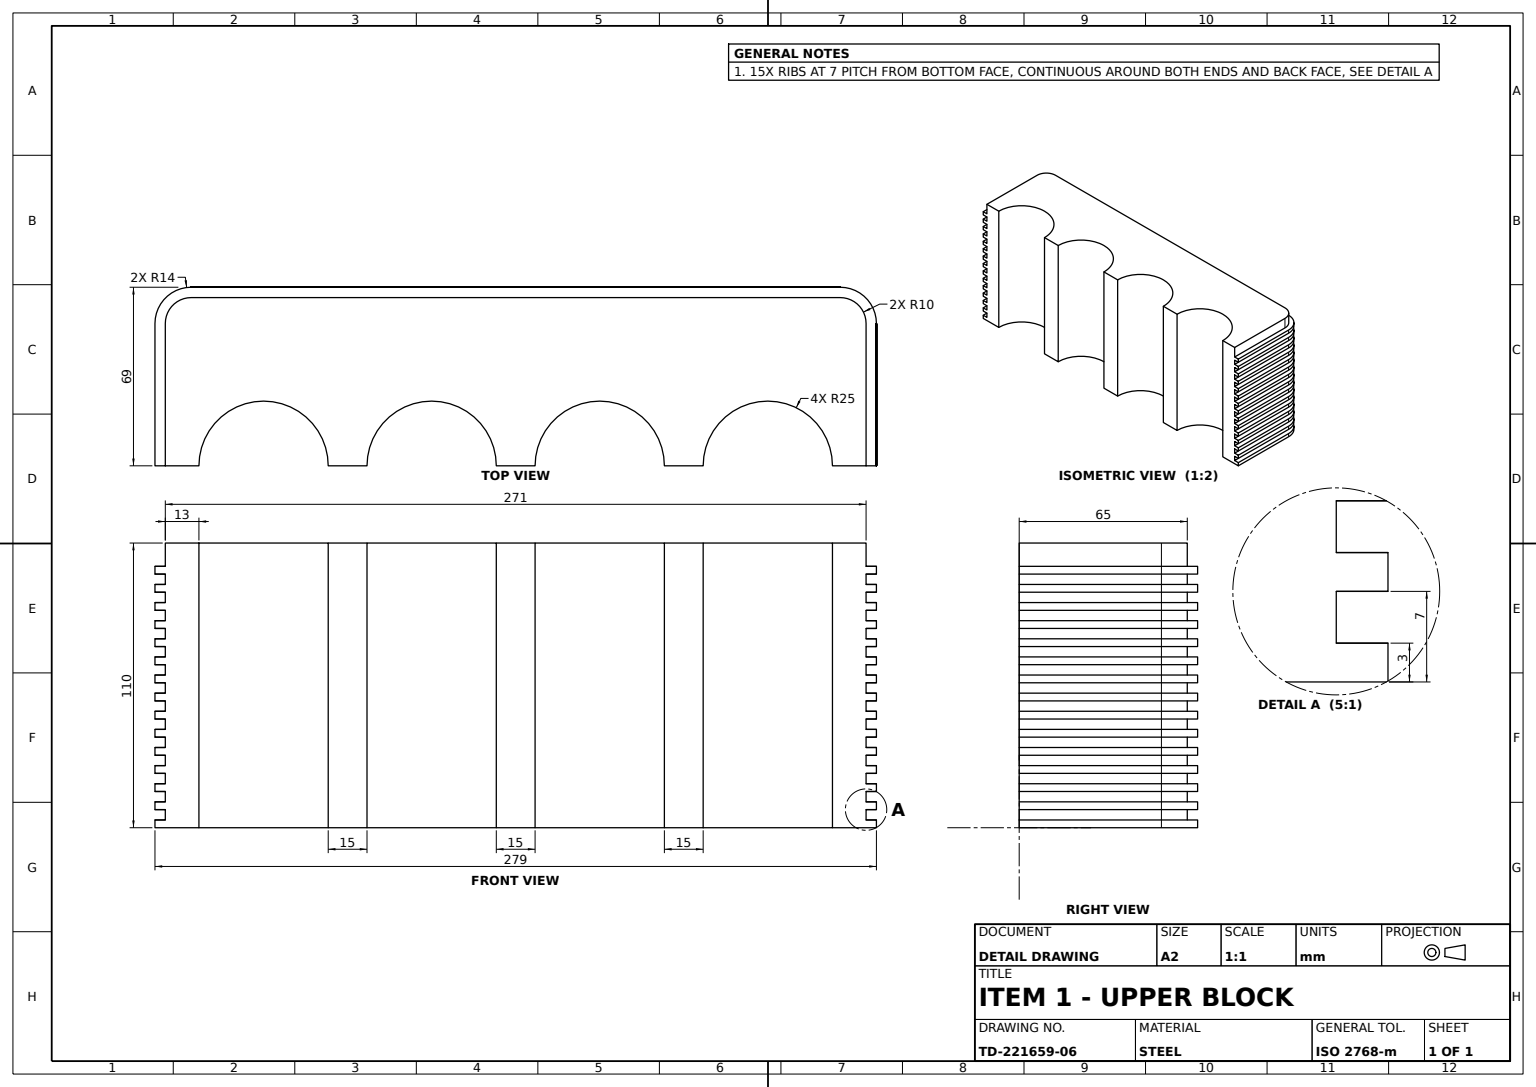
solid
v1 (0,28,-55)
v2 (0,24,-55)
e1 v1 v2 LINE
v3 (10,28,-65)
e2 v1 v3 CIRCLE(AX(P(10,28,-55),D(0,-1,0),D(0,0,1)),10)
v4 (10,24,-65)
e3 v3 v4 LINE
e4 v2 v4 CIRCLE(AX(P(10,24,-55),D(0,-1,0),D(0,0,1)),10)
face CYL(AX(P(10,110,-55),D(0,-1,0),D(0,0,-1)),10) [-e1 e2 e3 -e4]
v5 (-4,49,0)
v6 (0,49,0)
e5 v5 v6 LINE
v7 (-4,49,-55)
e6 v7 v5 LINE
v8 (10,49,-69)
e7 v8 v7 CIRCLE(AX(P(10,49,-55),D(0,1,0),D(0,0,1)),14)
v9 (261,49,-69)
e8 v9 v8 LINE
v10 (275,49,-55)
e9 v10 v9 CIRCLE(AX(P(261,49,-55),D(0,1,0),D(0,0,1)),14)
v11 (275,49,0)
e10 v11 v10 LINE
v12 (271,49,0)
e11 v12 v11 LINE
v13 (271,49,-55)
e12 v13 v12 LINE
v14 (261,49,-65)
e13 v14 v13 CIRCLE(AX(P(261,49,-55),D(0,-1,0),D(0,0,1)),10)
v15 (10,49,-65)
e14 v15 v14 LINE
v16 (0,49,-55)
e15 v16 v15 CIRCLE(AX(P(10,49,-55),D(0,-1,0),D(0,0,1)),10)
e16 v6 v16 LINE
face PLANE(AX(P(10,49,-55),D(0,1,0),D(0,0,1))) rev [-e5 -e6 -e7 -e8 -e9 -e10 -e11 -e12 -e13 -e14 -e15 -e16]
v17 (275,94,-55)
v18 (275,91,-55)
e17 v17 v18 LINE
v19 (275,94,0)
e18 v19 v17 LINE
v20 (275,91,0)
e19 v19 v20 LINE
e20 v20 v18 LINE
face PLANE(AX(P(275,94,0),D(-1,0,0),D(0,0,1))) rev [-e17 -e18 e19 e20]
v21 (271,80,-55)
v22 (271,80,0)
e21 v21 v22 LINE
v23 (271,84,-55)
e22 v23 v21 LINE
v24 (271,84,0)
e23 v23 v24 LINE
e24 v24 v22 LINE
face PLANE(AX(P(271,110,0),D(-1,0,0),D(0,0,1))) rev [-e21 -e22 e23 e24]
v25 (-4,10,-55)
v26 (-4,7,-55)
e25 v25 v26 LINE
v27 (10,10,-69)
e26 v27 v25 CIRCLE(AX(P(10,10,-55),D(0,1,0),D(0,0,1)),14)
v28 (10,7,-69)
e27 v27 v28 LINE
e28 v28 v26 CIRCLE(AX(P(10,7,-55),D(0,1,0),D(0,0,1)),14)
face CYL(AX(P(10,10,-55),D(0,-1,0),D(0,0,-1)),14) [-e25 -e26 e27 e28]
v29 (275,10,-55)
v30 (275,7,-55)
e29 v29 v30 LINE
v31 (275,10,0)
e30 v31 v29 LINE
v32 (275,7,0)
e31 v31 v32 LINE
e32 v32 v30 LINE
face PLANE(AX(P(275,10,0),D(-1,0,0),D(0,0,1))) rev [-e29 -e30 e31 e32]
v33 (10,24,-69)
v34 (10,21,-69)
e33 v33 v34 LINE
v35 (261,24,-69)
e34 v35 v33 LINE
v36 (261,21,-69)
e35 v35 v36 LINE
e36 v36 v34 LINE
face PLANE(AX(P(261,24,-69),D(0,0,1),D(1,0,0))) rev [-e33 -e34 e35 e36]
v37 (10,3,-69)
v38 (-4,3,-55)
e37 v37 v38 CIRCLE(AX(P(10,3,-55),D(0,1,0),D(0,0,1)),14)
v39 (10,0,-69)
e38 v37 v39 LINE
v40 (-4,0,-55)
e39 v39 v40 CIRCLE(AX(P(10,0,-55),D(0,1,0),D(0,0,1)),14)
e40 v38 v40 LINE
face CYL(AX(P(10,3,-55),D(0,-1,0),D(0,0,-1)),14) [-e37 e38 e39 -e40]
v41 (10,52,-69)
v42 (-4,52,-55)
e41 v41 v42 CIRCLE(AX(P(10,52,-55),D(0,1,0),D(0,0,1)),14)
e42 v41 v8 LINE
e43 v42 v7 LINE
face CYL(AX(P(10,52,-55),D(0,-1,0),D(0,0,-1)),14) [-e41 e42 e7 -e43]
v43 (0,73,0)
v44 (0,73,-55)
e44 v43 v44 LINE
v45 (0,77,0)
e45 v45 v43 LINE
v46 (0,77,-55)
e46 v45 v46 LINE
e47 v46 v44 LINE
face PLANE(AX(P(0,110,0),D(1,0,0),D(0,0,-1))) rev [-e44 -e45 e46 e47]
v47 (0,42,-55)
v48 (10,42,-65)
e48 v47 v48 CIRCLE(AX(P(10,42,-55),D(0,-1,0),D(0,0,1)),10)
v49 (10,38,-65)
e49 v48 v49 LINE
v50 (0,38,-55)
e50 v50 v49 CIRCLE(AX(P(10,38,-55),D(0,-1,0),D(0,0,1)),10)
e51 v47 v50 LINE
face CYL(AX(P(10,110,-55),D(0,-1,0),D(0,0,-1)),10) [e48 e49 -e50 -e51]
v51 (261,45,-65)
v52 (271,45,-55)
e52 v51 v52 CIRCLE(AX(P(261,45,-55),D(0,-1,0),D(0,0,1)),10)
v53 (271,45,0)
e53 v52 v53 LINE
v54 (275,45,0)
e54 v53 v54 LINE
v55 (275,45,-55)
e55 v54 v55 LINE
v56 (261,45,-69)
e56 v55 v56 CIRCLE(AX(P(261,45,-55),D(0,1,0),D(0,0,1)),14)
v57 (10,45,-69)
e57 v56 v57 LINE
v58 (-4,45,-55)
e58 v57 v58 CIRCLE(AX(P(10,45,-55),D(0,1,0),D(0,0,1)),14)
v59 (-4,45,0)
e59 v58 v59 LINE
v60 (0,45,0)
e60 v59 v60 LINE
v61 (0,45,-55)
e61 v60 v61 LINE
v62 (10,45,-65)
e62 v61 v62 CIRCLE(AX(P(10,45,-55),D(0,-1,0),D(0,0,1)),10)
e63 v62 v51 LINE
face PLANE(AX(P(10,45,-55),D(0,1,0),D(0,0,1))) [e52 e53 e54 e55 e56 e57 e58 e59 e60 e61 e62 e63]
v63 (261,91,-65)
v64 (271,91,-55)
e64 v63 v64 CIRCLE(AX(P(261,91,-55),D(0,-1,0),D(0,0,1)),10)
v65 (10,91,-65)
e65 v65 v63 LINE
v66 (0,91,-55)
e66 v66 v65 CIRCLE(AX(P(10,91,-55),D(0,-1,0),D(0,0,1)),10)
v67 (0,91,0)
e67 v67 v66 LINE
v68 (-4,91,0)
e68 v68 v67 LINE
v69 (-4,91,-55)
e69 v69 v68 LINE
v70 (10,91,-69)
e70 v70 v69 CIRCLE(AX(P(10,91,-55),D(0,1,0),D(0,0,1)),14)
v71 (261,91,-69)
e71 v71 v70 LINE
e72 v18 v71 CIRCLE(AX(P(261,91,-55),D(0,1,0),D(0,0,1)),14)
v72 (271,91,0)
e73 v72 v20 LINE
e74 v64 v72 LINE
face PLANE(AX(P(10,91,-55),D(0,1,0),D(0,0,1))) rev [-e64 -e65 -e66 -e67 -e68 -e69 -e70 -e71 -e72 -e20 -e73 -e74]
v73 (261,94,-69)
e75 v17 v73 CIRCLE(AX(P(261,94,-55),D(0,1,0),D(0,0,1)),14)
e76 v73 v71 LINE
face CYL(AX(P(261,94,-55),D(0,-1,0),D(0,0,-1)),14) [-e75 e17 e72 -e76]
v74 (261,101,-69)
v75 (261,98,-69)
e77 v74 v75 LINE
v76 (10,98,-69)
e78 v75 v76 LINE
v77 (10,101,-69)
e79 v77 v76 LINE
e80 v74 v77 LINE
face PLANE(AX(P(261,101,-69),D(0,0,1),D(1,0,0))) rev [e77 e78 -e79 -e80]
v78 (233,110,-25)
v79 (233,0,-25)
e81 v78 v79 LINE
v80 (208,110,0)
e82 v80 v78 CIRCLE(AX(P(233,110,0),D(0,-1,0),D(0,0,1)),25)
v81 (208,0,0)
e83 v80 v81 LINE
e84 v81 v79 CIRCLE(AX(P(233,0,0),D(0,-1,0),D(0,0,1)),25)
face CYL(AX(P(233,110,0),D(0,-1,0),D(0,0,-1)),25) rev [-e81 -e82 e83 e84]
v82 (10,56,-69)
v83 (-4,56,-55)
e85 v82 v83 CIRCLE(AX(P(10,56,-55),D(0,1,0),D(0,0,1)),14)
v84 (-4,59,-55)
e86 v84 v83 LINE
v85 (10,59,-69)
e87 v85 v84 CIRCLE(AX(P(10,59,-55),D(0,1,0),D(0,0,1)),14)
e88 v85 v82 LINE
face CYL(AX(P(10,59,-55),D(0,-1,0),D(0,0,-1)),14) [e85 -e86 -e87 e88]
v86 (0,31,-55)
v87 (10,31,-65)
e89 v86 v87 CIRCLE(AX(P(10,31,-55),D(0,-1,0),D(0,0,1)),10)
v88 (0,35,-55)
e90 v88 v86 LINE
v89 (10,35,-65)
e91 v88 v89 CIRCLE(AX(P(10,35,-55),D(0,-1,0),D(0,0,1)),10)
e92 v89 v87 LINE
face CYL(AX(P(10,110,-55),D(0,-1,0),D(0,0,-1)),10) [-e89 -e90 e91 e92]
v90 (271,35,-55)
v91 (271,31,-55)
e93 v90 v91 LINE
v92 (261,31,-65)
e94 v92 v91 CIRCLE(AX(P(261,31,-55),D(0,-1,0),D(0,0,1)),10)
v93 (261,35,-65)
e95 v93 v92 LINE
e96 v93 v90 CIRCLE(AX(P(261,35,-55),D(0,-1,0),D(0,0,1)),10)
face CYL(AX(P(261,110,-55),D(0,-1,0),D(0,0,-1)),10) [e93 -e94 -e95 e96]
v94 (261,52,-69)
e97 v94 v9 LINE
e98 v94 v41 LINE
face PLANE(AX(P(261,52,-69),D(0,0,1),D(1,0,0))) rev [e97 e8 -e42 -e98]
v95 (0,3,0)
v96 (0,3,-55)
e99 v95 v96 LINE
v97 (0,7,0)
e100 v97 v95 LINE
v98 (0,7,-55)
e101 v97 v98 LINE
e102 v98 v96 LINE
face PLANE(AX(P(0,110,0),D(1,0,0),D(0,0,-1))) rev [-e99 -e100 e101 e102]
v99 (275,80,0)
v100 (275,77,0)
e103 v99 v100 LINE
v101 (275,77,-55)
e104 v100 v101 LINE
v102 (275,80,-55)
e105 v102 v101 LINE
e106 v99 v102 LINE
face PLANE(AX(P(275,80,0),D(-1,0,0),D(0,0,1))) rev [e103 e104 -e105 -e106]
v103 (261,24,-65)
v104 (271,24,-55)
e107 v103 v104 CIRCLE(AX(P(261,24,-55),D(0,-1,0),D(0,0,1)),10)
v105 (261,28,-65)
e108 v105 v103 LINE
v106 (271,28,-55)
e109 v105 v106 CIRCLE(AX(P(261,28,-55),D(0,-1,0),D(0,0,1)),10)
e110 v106 v104 LINE
face CYL(AX(P(261,110,-55),D(0,-1,0),D(0,0,-1)),10) [-e107 -e108 e109 e110]
v107 (10,31,-69)
v108 (-4,31,-55)
e111 v107 v108 CIRCLE(AX(P(10,31,-55),D(0,1,0),D(0,0,1)),14)
v109 (10,28,-69)
e112 v107 v109 LINE
v110 (-4,28,-55)
e113 v109 v110 CIRCLE(AX(P(10,28,-55),D(0,1,0),D(0,0,1)),14)
e114 v108 v110 LINE
face CYL(AX(P(10,31,-55),D(0,-1,0),D(0,0,-1)),14) [-e111 e112 e113 -e114]
v111 (261,87,-69)
v112 (261,84,-69)
e115 v111 v112 LINE
v113 (10,84,-69)
e116 v112 v113 LINE
v114 (10,87,-69)
e117 v114 v113 LINE
e118 v111 v114 LINE
face PLANE(AX(P(261,87,-69),D(0,0,1),D(1,0,0))) rev [e115 e116 -e117 -e118]
v115 (63,110,0)
v116 (63,0,0)
e119 v115 v116 LINE
v117 (38,110,-25)
e120 v117 v115 CIRCLE(AX(P(38,110,0),D(0,-1,0),D(0,0,-1)),25)
v118 (38,0,-25)
e121 v117 v118 LINE
e122 v118 v116 CIRCLE(AX(P(38,0,0),D(0,-1,0),D(0,0,-1)),25)
face CYL(AX(P(38,110,0),D(0,-1,0),D(0,0,-1)),25) rev [-e119 -e120 e121 e122]
v119 (275,24,-55)
e123 v119 v35 CIRCLE(AX(P(261,24,-55),D(0,1,0),D(0,0,1)),14)
v120 (275,21,-55)
e124 v119 v120 LINE
e125 v120 v36 CIRCLE(AX(P(261,21,-55),D(0,1,0),D(0,0,1)),14)
face CYL(AX(P(261,24,-55),D(0,-1,0),D(0,0,-1)),14) [-e123 e124 e125 -e35]
v121 (78,110,0)
v122 (78,0,0)
e126 v121 v122 LINE
e127 v115 v121 LINE
e128 v116 v122 LINE
face PLANE(AX(P(63,110,0),D(0,0,-1),D(-1,0,0))) rev [-e126 -e127 e119 e128]
v123 (10,70,-65)
v124 (10,66,-65)
e129 v123 v124 LINE
v125 (0,66,-55)
e130 v125 v124 CIRCLE(AX(P(10,66,-55),D(0,-1,0),D(0,0,1)),10)
v126 (0,70,-55)
e131 v126 v125 LINE
e132 v126 v123 CIRCLE(AX(P(10,70,-55),D(0,-1,0),D(0,0,1)),10)
face CYL(AX(P(10,110,-55),D(0,-1,0),D(0,0,-1)),10) [e129 -e130 -e131 e132]
v127 (275,21,0)
e133 v127 v120 LINE
v128 (275,24,0)
e134 v128 v119 LINE
e135 v128 v127 LINE
face PLANE(AX(P(275,24,0),D(-1,0,0),D(0,0,1))) rev [e133 -e124 -e134 e135]
v129 (-4,87,-55)
v130 (-4,84,-55)
e136 v129 v130 LINE
v131 (-4,84,0)
e137 v130 v131 LINE
v132 (-4,87,0)
e138 v132 v131 LINE
e139 v129 v132 LINE
face PLANE(AX(P(-4,87,-55),D(1,0,0),D(0,0,-1))) rev [e136 e137 -e138 -e139]
v133 (271,56,-55)
v134 (271,52,-55)
e140 v133 v134 LINE
v135 (271,56,0)
e141 v133 v135 LINE
v136 (271,52,0)
e142 v135 v136 LINE
e143 v134 v136 LINE
face PLANE(AX(P(271,110,0),D(-1,0,0),D(0,0,1))) rev [-e140 e141 e142 -e143]
v137 (10,94,-69)
v138 (-4,94,-55)
e144 v137 v138 CIRCLE(AX(P(10,94,-55),D(0,1,0),D(0,0,1)),14)
e145 v137 v70 LINE
e146 v138 v69 LINE
face CYL(AX(P(10,94,-55),D(0,-1,0),D(0,0,-1)),14) [-e144 e145 e70 -e146]
v139 (275,42,-55)
v140 (261,42,-69)
e147 v139 v140 CIRCLE(AX(P(261,42,-55),D(0,1,0),D(0,0,1)),14)
e148 v56 v140 LINE
e149 v55 v139 LINE
face CYL(AX(P(261,45,-55),D(0,-1,0),D(0,0,-1)),14) [e147 -e148 -e56 e149]
v141 (275,31,0)
v142 (275,28,0)
e150 v141 v142 LINE
v143 (275,28,-55)
e151 v142 v143 LINE
v144 (275,31,-55)
e152 v144 v143 LINE
e153 v141 v144 LINE
face PLANE(AX(P(275,31,0),D(-1,0,0),D(0,0,1))) rev [e150 e151 -e152 -e153]
v145 (10,63,-65)
v146 (10,59,-65)
e154 v145 v146 LINE
v147 (261,63,-65)
e155 v145 v147 LINE
v148 (261,59,-65)
e156 v147 v148 LINE
e157 v146 v148 LINE
face PLANE(AX(P(10,110,-65),D(0,0,1),D(1,0,0))) rev [-e154 e155 e156 -e157]
v149 (275,0,0)
v150 (275,0,-55)
e158 v149 v150 LINE
v151 (275,3,-55)
e159 v151 v150 LINE
v152 (275,3,0)
e160 v152 v151 LINE
e161 v152 v149 LINE
face PLANE(AX(P(275,3,0),D(-1,0,0),D(0,0,1))) rev [e158 -e159 -e160 e161]
v153 (275,17,0)
v154 (275,17,-55)
e162 v153 v154 LINE
v155 (275,14,0)
e163 v153 v155 LINE
v156 (275,14,-55)
e164 v155 v156 LINE
e165 v154 v156 LINE
face PLANE(AX(P(275,17,0),D(-1,0,0),D(0,0,1))) rev [-e162 e163 e164 -e165]
v157 (168,110,-25)
v158 (168,0,-25)
e166 v157 v158 LINE
v159 (143,110,0)
e167 v159 v157 CIRCLE(AX(P(168,110,0),D(0,-1,0),D(0,0,1)),25)
v160 (143,0,0)
e168 v159 v160 LINE
e169 v160 v158 CIRCLE(AX(P(168,0,0),D(0,-1,0),D(0,0,1)),25)
face CYL(AX(P(168,110,0),D(0,-1,0),D(0,0,-1)),25) rev [-e166 -e167 e168 e169]
v161 (261,59,-69)
v162 (261,56,-69)
e170 v161 v162 LINE
v163 (275,59,-55)
e171 v163 v161 CIRCLE(AX(P(261,59,-55),D(0,1,0),D(0,0,1)),14)
v164 (275,56,-55)
e172 v163 v164 LINE
e173 v164 v162 CIRCLE(AX(P(261,56,-55),D(0,1,0),D(0,0,1)),14)
face CYL(AX(P(261,59,-55),D(0,-1,0),D(0,0,-1)),14) [-e170 -e171 e172 e173]
v165 (-4,3,0)
e174 v38 v165 LINE
e175 v165 v95 LINE
v166 (10,3,-65)
e176 v96 v166 CIRCLE(AX(P(10,3,-55),D(0,-1,0),D(0,0,1)),10)
v167 (261,3,-65)
e177 v166 v167 LINE
v168 (271,3,-55)
e178 v167 v168 CIRCLE(AX(P(261,3,-55),D(0,-1,0),D(0,0,1)),10)
v169 (271,3,0)
e179 v168 v169 LINE
e180 v169 v152 LINE
v170 (261,3,-69)
e181 v151 v170 CIRCLE(AX(P(261,3,-55),D(0,1,0),D(0,0,1)),14)
e182 v170 v37 LINE
face PLANE(AX(P(10,3,-55),D(0,1,0),D(0,0,1))) [e37 e174 e175 e99 e176 e177 e178 e179 e180 e160 e181 e182]
v171 (271,87,0)
e183 v72 v171 LINE
v172 (271,87,-55)
e184 v172 v171 LINE
e185 v64 v172 LINE
face PLANE(AX(P(271,110,0),D(-1,0,0),D(0,0,1))) rev [e183 -e184 -e185 e74]
v173 (261,28,-69)
e186 v143 v173 CIRCLE(AX(P(261,28,-55),D(0,1,0),D(0,0,1)),14)
v174 (261,31,-69)
e187 v174 v173 LINE
e188 v144 v174 CIRCLE(AX(P(261,31,-55),D(0,1,0),D(0,0,1)),14)
face CYL(AX(P(261,31,-55),D(0,-1,0),D(0,0,-1)),14) [e186 -e187 -e188 e152]
v175 (261,14,-65)
v176 (261,10,-65)
e189 v175 v176 LINE
v177 (10,10,-65)
e190 v177 v176 LINE
v178 (10,14,-65)
e191 v178 v177 LINE
e192 v178 v175 LINE
face PLANE(AX(P(10,110,-65),D(0,0,1),D(1,0,0))) rev [e189 -e190 -e191 e192]
v179 (0,56,-55)
v180 (10,56,-65)
e193 v179 v180 CIRCLE(AX(P(10,56,-55),D(0,-1,0),D(0,0,1)),10)
v181 (10,52,-65)
e194 v180 v181 LINE
v182 (0,52,-55)
e195 v182 v181 CIRCLE(AX(P(10,52,-55),D(0,-1,0),D(0,0,1)),10)
e196 v179 v182 LINE
face CYL(AX(P(10,110,-55),D(0,-1,0),D(0,0,-1)),10) [e193 e194 -e195 -e196]
v183 (275,59,0)
e197 v183 v163 LINE
v184 (275,56,0)
e198 v183 v184 LINE
e199 v184 v164 LINE
face PLANE(AX(P(275,59,0),D(-1,0,0),D(0,0,1))) rev [-e172 -e197 e198 e199]
v185 (10,21,-65)
v186 (261,21,-65)
e200 v185 v186 LINE
v187 (0,21,-55)
e201 v187 v185 CIRCLE(AX(P(10,21,-55),D(0,-1,0),D(0,0,1)),10)
v188 (0,21,0)
e202 v188 v187 LINE
v189 (-4,21,0)
e203 v189 v188 LINE
v190 (-4,21,-55)
e204 v190 v189 LINE
e205 v34 v190 CIRCLE(AX(P(10,21,-55),D(0,1,0),D(0,0,1)),14)
v191 (271,21,0)
e206 v191 v127 LINE
v192 (271,21,-55)
e207 v192 v191 LINE
e208 v186 v192 CIRCLE(AX(P(261,21,-55),D(0,-1,0),D(0,0,1)),10)
face PLANE(AX(P(10,21,-55),D(0,1,0),D(0,0,1))) rev [-e200 -e201 -e202 -e203 -e204 -e205 -e36 -e125 -e133 -e206 -e207 -e208]
v193 (-4,28,0)
e209 v110 v193 LINE
v194 (-4,31,0)
e210 v194 v193 LINE
e211 v108 v194 LINE
face PLANE(AX(P(-4,31,-55),D(1,0,0),D(0,0,-1))) rev [e209 -e210 -e211 e114]
v195 (271,42,-55)
v196 (271,38,-55)
e212 v195 v196 LINE
v197 (261,38,-65)
e213 v197 v196 CIRCLE(AX(P(261,38,-55),D(0,-1,0),D(0,0,1)),10)
v198 (261,42,-65)
e214 v198 v197 LINE
e215 v198 v195 CIRCLE(AX(P(261,42,-55),D(0,-1,0),D(0,0,1)),10)
face CYL(AX(P(261,110,-55),D(0,-1,0),D(0,0,-1)),10) [e212 -e213 -e214 e215]
v199 (261,66,-65)
e216 v124 v199 LINE
v200 (261,70,-65)
e217 v123 v200 LINE
e218 v200 v199 LINE
face PLANE(AX(P(10,110,-65),D(0,0,1),D(1,0,0))) rev [-e216 -e129 e217 e218]
v201 (275,73,-55)
v202 (261,73,-69)
e219 v201 v202 CIRCLE(AX(P(261,73,-55),D(0,1,0),D(0,0,1)),14)
v203 (275,70,-55)
e220 v201 v203 LINE
v204 (261,70,-69)
e221 v203 v204 CIRCLE(AX(P(261,70,-55),D(0,1,0),D(0,0,1)),14)
e222 v202 v204 LINE
face CYL(AX(P(261,73,-55),D(0,-1,0),D(0,0,-1)),14) [-e219 e220 e221 -e222]
v205 (10,42,-69)
e223 v140 v205 LINE
v206 (275,42,0)
e224 v206 v139 LINE
v207 (271,42,0)
e225 v207 v206 LINE
e226 v195 v207 LINE
e227 v48 v198 LINE
v208 (0,42,0)
e228 v208 v47 LINE
v209 (-4,42,0)
e229 v209 v208 LINE
v210 (-4,42,-55)
e230 v210 v209 LINE
e231 v205 v210 CIRCLE(AX(P(10,42,-55),D(0,1,0),D(0,0,1)),14)
face PLANE(AX(P(10,42,-55),D(0,1,0),D(0,0,1))) rev [-e223 -e147 -e224 -e225 -e226 -e215 -e227 -e48 -e228 -e229 -e230 -e231]
e232 v58 v210 LINE
e233 v59 v209 LINE
face PLANE(AX(P(-4,45,-55),D(1,0,0),D(0,0,-1))) rev [-e59 e232 e230 -e233]
v211 (271,7,-55)
e234 v211 v168 LINE
v212 (271,7,0)
e235 v211 v212 LINE
e236 v212 v169 LINE
face PLANE(AX(P(271,110,0),D(-1,0,0),D(0,0,1))) rev [-e234 e235 e236 -e179]
v213 (0,110,-55)
v214 (0,110,0)
e237 v213 v214 LINE
v215 (13,110,0)
e238 v214 v215 LINE
e239 v215 v117 CIRCLE(AX(P(38,110,0),D(0,-1,0),D(0,0,-1)),25)
v216 (103,110,-25)
e240 v121 v216 CIRCLE(AX(P(103,110,0),D(0,-1,0),D(0,0,-1)),25)
v217 (128,110,0)
e241 v216 v217 CIRCLE(AX(P(103,110,0),D(0,-1,0),D(0,0,-1)),25)
e242 v217 v159 LINE
v218 (193,110,0)
e243 v157 v218 CIRCLE(AX(P(168,110,0),D(0,-1,0),D(0,0,1)),25)
e244 v218 v80 LINE
v219 (258,110,0)
e245 v78 v219 CIRCLE(AX(P(233,110,0),D(0,-1,0),D(0,0,1)),25)
v220 (271,110,0)
e246 v219 v220 LINE
v221 (271,110,-55)
e247 v220 v221 LINE
v222 (261,110,-65)
e248 v221 v222 CIRCLE(AX(P(261,110,-55),D(0,1,0),D(0,0,-1)),10)
v223 (10,110,-65)
e249 v222 v223 LINE
e250 v223 v213 CIRCLE(AX(P(10,110,-55),D(0,1,0),D(0,0,-1)),10)
face PLANE(AX(P(10,110,-55),D(0,-1,0),D(0,0,-1))) rev [e237 e238 e239 e120 e127 e240 e241 e242 e167 e243 e244 e82 e245 e246 e247 e248 e249 e250]
v224 (261,73,-65)
v225 (271,73,-55)
e251 v224 v225 CIRCLE(AX(P(261,73,-55),D(0,-1,0),D(0,0,1)),10)
v226 (261,77,-65)
e252 v226 v224 LINE
v227 (271,77,-55)
e253 v226 v227 CIRCLE(AX(P(261,77,-55),D(0,-1,0),D(0,0,1)),10)
e254 v227 v225 LINE
face CYL(AX(P(261,110,-55),D(0,-1,0),D(0,0,-1)),10) [-e251 -e252 e253 e254]
v228 (0,87,-55)
v229 (10,87,-65)
e255 v228 v229 CIRCLE(AX(P(10,87,-55),D(0,-1,0),D(0,0,1)),10)
e256 v66 v228 LINE
e257 v65 v229 LINE
face CYL(AX(P(10,110,-55),D(0,-1,0),D(0,0,-1)),10) [-e255 -e256 e66 e257]
v230 (-4,73,-55)
v231 (-4,70,-55)
e258 v230 v231 LINE
v232 (10,73,-69)
e259 v232 v230 CIRCLE(AX(P(10,73,-55),D(0,1,0),D(0,0,1)),14)
v233 (10,70,-69)
e260 v232 v233 LINE
e261 v233 v231 CIRCLE(AX(P(10,70,-55),D(0,1,0),D(0,0,1)),14)
face CYL(AX(P(10,73,-55),D(0,-1,0),D(0,0,-1)),14) [-e258 -e259 e260 e261]
e262 v57 v205 LINE
face PLANE(AX(P(261,45,-69),D(0,0,1),D(1,0,0))) rev [e223 -e262 -e57 e148]
v234 (0,94,0)
v235 (0,94,-55)
e263 v234 v235 LINE
v236 (0,98,0)
e264 v236 v234 LINE
v237 (0,98,-55)
e265 v236 v237 LINE
e266 v237 v235 LINE
face PLANE(AX(P(0,110,0),D(1,0,0),D(0,0,-1))) rev [-e263 -e264 e265 e266]
v238 (-4,70,0)
e267 v231 v238 LINE
v239 (-4,73,0)
e268 v239 v238 LINE
e269 v230 v239 LINE
face PLANE(AX(P(-4,73,-55),D(1,0,0),D(0,0,-1))) rev [e258 e267 -e268 -e269]
e270 v16 v61 LINE
e271 v15 v62 LINE
face CYL(AX(P(10,110,-55),D(0,-1,0),D(0,0,-1)),10) [-e62 -e270 e15 e271]
v240 (271,17,-55)
v241 (271,17,0)
e272 v240 v241 LINE
e273 v192 v240 LINE
e274 v191 v241 LINE
face PLANE(AX(P(271,110,0),D(-1,0,0),D(0,0,1))) rev [-e272 -e273 e207 e274]
v242 (-4,35,0)
v243 (0,35,0)
e275 v242 v243 LINE
v244 (-4,35,-55)
e276 v244 v242 LINE
v245 (10,35,-69)
e277 v245 v244 CIRCLE(AX(P(10,35,-55),D(0,1,0),D(0,0,1)),14)
v246 (261,35,-69)
e278 v246 v245 LINE
v247 (275,35,-55)
e279 v247 v246 CIRCLE(AX(P(261,35,-55),D(0,1,0),D(0,0,1)),14)
v248 (275,35,0)
e280 v248 v247 LINE
v249 (271,35,0)
e281 v249 v248 LINE
e282 v90 v249 LINE
e283 v89 v93 LINE
e284 v243 v88 LINE
face PLANE(AX(P(10,35,-55),D(0,1,0),D(0,0,1))) rev [-e275 -e276 -e277 -e278 -e279 -e280 -e281 -e282 -e96 -e283 -e91 -e284]
v250 (0,101,-55)
e285 v213 v250 LINE
v251 (0,101,0)
e286 v251 v250 LINE
e287 v214 v251 LINE
face PLANE(AX(P(0,110,0),D(1,0,0),D(0,0,-1))) rev [-e237 e285 -e286 -e287]
v252 (10,17,-69)
v253 (-4,17,-55)
e288 v252 v253 CIRCLE(AX(P(10,17,-55),D(0,1,0),D(0,0,1)),14)
v254 (-4,17,0)
e289 v253 v254 LINE
v255 (0,17,0)
e290 v254 v255 LINE
v256 (0,17,-55)
e291 v255 v256 LINE
v257 (10,17,-65)
e292 v256 v257 CIRCLE(AX(P(10,17,-55),D(0,-1,0),D(0,0,1)),10)
v258 (261,17,-65)
e293 v257 v258 LINE
e294 v258 v240 CIRCLE(AX(P(261,17,-55),D(0,-1,0),D(0,0,1)),10)
e295 v241 v153 LINE
v259 (261,17,-69)
e296 v154 v259 CIRCLE(AX(P(261,17,-55),D(0,1,0),D(0,0,1)),14)
e297 v259 v252 LINE
face PLANE(AX(P(10,17,-55),D(0,1,0),D(0,0,1))) [e288 e289 e290 e291 e292 e293 e294 e272 e295 e162 e296 e297]
v260 (0,10,-55)
e298 v260 v177 CIRCLE(AX(P(10,10,-55),D(0,-1,0),D(0,0,1)),10)
v261 (0,14,-55)
e299 v261 v260 LINE
e300 v261 v178 CIRCLE(AX(P(10,14,-55),D(0,-1,0),D(0,0,1)),10)
face CYL(AX(P(10,110,-55),D(0,-1,0),D(0,0,-1)),10) [e191 -e298 -e299 e300]
v262 (275,98,-55)
e301 v262 v75 CIRCLE(AX(P(261,98,-55),D(0,1,0),D(0,0,1)),14)
v263 (275,101,-55)
e302 v263 v74 CIRCLE(AX(P(261,101,-55),D(0,1,0),D(0,0,1)),14)
e303 v263 v262 LINE
face CYL(AX(P(261,101,-55),D(0,-1,0),D(0,0,-1)),14) [e301 -e77 -e302 e303]
v264 (261,14,-69)
v265 (10,14,-69)
e304 v264 v265 LINE
e305 v252 v265 LINE
e306 v259 v264 LINE
face PLANE(AX(P(261,17,-69),D(0,0,1),D(1,0,0))) rev [e304 -e305 -e297 e306]
v266 (261,94,-65)
v267 (271,94,-55)
e307 v266 v267 CIRCLE(AX(P(261,94,-55),D(0,-1,0),D(0,0,1)),10)
v268 (261,98,-65)
e308 v268 v266 LINE
v269 (271,98,-55)
e309 v268 v269 CIRCLE(AX(P(261,98,-55),D(0,-1,0),D(0,0,1)),10)
e310 v269 v267 LINE
face CYL(AX(P(261,110,-55),D(0,-1,0),D(0,0,-1)),10) [-e307 -e308 e309 e310]
e311 v202 v232 LINE
e312 v204 v233 LINE
face PLANE(AX(P(261,73,-69),D(0,0,1),D(1,0,0))) rev [-e311 e222 e312 -e260]
v270 (-4,38,-55)
e313 v270 v244 LINE
v271 (10,38,-69)
e314 v271 v270 CIRCLE(AX(P(10,38,-55),D(0,1,0),D(0,0,1)),14)
e315 v271 v245 LINE
face CYL(AX(P(10,38,-55),D(0,-1,0),D(0,0,-1)),14) [-e313 -e314 e315 e277]
e316 v161 v85 LINE
v272 (-4,59,0)
e317 v84 v272 LINE
v273 (0,59,0)
e318 v272 v273 LINE
v274 (0,59,-55)
e319 v273 v274 LINE
e320 v274 v146 CIRCLE(AX(P(10,59,-55),D(0,-1,0),D(0,0,1)),10)
v275 (271,59,-55)
e321 v148 v275 CIRCLE(AX(P(261,59,-55),D(0,-1,0),D(0,0,1)),10)
v276 (271,59,0)
e322 v275 v276 LINE
e323 v276 v183 LINE
face PLANE(AX(P(10,59,-55),D(0,1,0),D(0,0,1))) [e316 e87 e317 e318 e319 e320 e157 e321 e322 e323 e197 e171]
v277 (-4,24,0)
e324 v277 v189 LINE
v278 (-4,24,-55)
e325 v278 v277 LINE
e326 v278 v190 LINE
face PLANE(AX(P(-4,24,-55),D(1,0,0),D(0,0,-1))) rev [e204 -e324 -e325 e326]
e327 v4 v103 LINE
v279 (271,24,0)
e328 v104 v279 LINE
e329 v279 v128 LINE
e330 v33 v278 CIRCLE(AX(P(10,24,-55),D(0,1,0),D(0,0,1)),14)
v280 (0,24,0)
e331 v277 v280 LINE
e332 v280 v2 LINE
face PLANE(AX(P(10,24,-55),D(0,1,0),D(0,0,1))) [e327 e107 e328 e329 e134 e123 e34 e330 e325 e331 e332 e4]
v281 (10,84,-65)
v282 (10,80,-65)
e333 v281 v282 LINE
v283 (0,80,-55)
e334 v283 v282 CIRCLE(AX(P(10,80,-55),D(0,-1,0),D(0,0,1)),10)
v284 (0,84,-55)
e335 v284 v283 LINE
e336 v284 v281 CIRCLE(AX(P(10,84,-55),D(0,-1,0),D(0,0,1)),10)
face CYL(AX(P(10,110,-55),D(0,-1,0),D(0,0,-1)),10) [e333 -e334 -e335 e336]
v285 (261,52,-65)
e337 v285 v134 CIRCLE(AX(P(261,52,-55),D(0,-1,0),D(0,0,1)),10)
v286 (261,56,-65)
e338 v286 v285 LINE
e339 v286 v133 CIRCLE(AX(P(261,56,-55),D(0,-1,0),D(0,0,1)),10)
face CYL(AX(P(261,110,-55),D(0,-1,0),D(0,0,-1)),10) [-e337 -e338 e339 e140]
v287 (193,0,0)
e340 v218 v287 LINE
e341 v158 v287 CIRCLE(AX(P(168,0,0),D(0,-1,0),D(0,0,1)),25)
face CYL(AX(P(168,110,0),D(0,-1,0),D(0,0,-1)),25) rev [-e340 -e243 e166 e341]
e342 v73 v137 LINE
face PLANE(AX(P(261,94,-69),D(0,0,1),D(1,0,0))) rev [-e145 -e342 e76 e71]
v288 (0,84,0)
e343 v131 v288 LINE
e344 v113 v130 CIRCLE(AX(P(10,84,-55),D(0,1,0),D(0,0,1)),14)
v289 (275,84,-55)
e345 v289 v112 CIRCLE(AX(P(261,84,-55),D(0,1,0),D(0,0,1)),14)
v290 (275,84,0)
e346 v290 v289 LINE
e347 v24 v290 LINE
v291 (261,84,-65)
e348 v291 v23 CIRCLE(AX(P(261,84,-55),D(0,-1,0),D(0,0,1)),10)
e349 v281 v291 LINE
e350 v288 v284 LINE
face PLANE(AX(P(10,84,-55),D(0,1,0),D(0,0,1))) rev [-e343 -e137 -e344 -e116 -e345 -e346 -e347 -e23 -e348 -e349 -e336 -e350]
v292 (271,14,0)
e351 v292 v155 LINE
v293 (271,14,-55)
e352 v293 v292 LINE
e353 v175 v293 CIRCLE(AX(P(261,14,-55),D(0,-1,0),D(0,0,1)),10)
v294 (0,14,0)
e354 v294 v261 LINE
v295 (-4,14,0)
e355 v295 v294 LINE
v296 (-4,14,-55)
e356 v296 v295 LINE
e357 v265 v296 CIRCLE(AX(P(10,14,-55),D(0,1,0),D(0,0,1)),14)
e358 v156 v264 CIRCLE(AX(P(261,14,-55),D(0,1,0),D(0,0,1)),14)
face PLANE(AX(P(10,14,-55),D(0,1,0),D(0,0,1))) rev [-e164 -e351 -e352 -e353 -e192 -e300 -e354 -e355 -e356 -e357 -e304 -e358]
v297 (10,73,-65)
e359 v297 v224 LINE
v298 (10,77,-65)
e360 v298 v297 LINE
e361 v298 v226 LINE
face PLANE(AX(P(10,110,-65),D(0,0,1),D(1,0,0))) rev [e252 -e359 -e360 e361]
v299 (0,80,0)
e362 v299 v283 LINE
v300 (261,80,-65)
e363 v282 v300 LINE
e364 v300 v21 CIRCLE(AX(P(261,80,-55),D(0,-1,0),D(0,0,1)),10)
e365 v22 v99 LINE
v301 (261,80,-69)
e366 v102 v301 CIRCLE(AX(P(261,80,-55),D(0,1,0),D(0,0,1)),14)
v302 (10,80,-69)
e367 v301 v302 LINE
v303 (-4,80,-55)
e368 v302 v303 CIRCLE(AX(P(10,80,-55),D(0,1,0),D(0,0,1)),14)
v304 (-4,80,0)
e369 v303 v304 LINE
e370 v304 v299 LINE
face PLANE(AX(P(10,80,-55),D(0,1,0),D(0,0,1))) [e362 e334 e363 e364 e21 e365 e106 e366 e367 e368 e369 e370]
e371 v291 v300 LINE
face PLANE(AX(P(10,110,-65),D(0,0,1),D(1,0,0))) rev [-e333 e349 e371 -e363]
v305 (275,52,-55)
e372 v305 v94 CIRCLE(AX(P(261,52,-55),D(0,1,0),D(0,0,1)),14)
e373 v305 v10 LINE
face CYL(AX(P(261,52,-55),D(0,-1,0),D(0,0,-1)),14) [-e97 -e372 e373 e9]
e374 v185 v257 LINE
e375 v186 v258 LINE
face PLANE(AX(P(10,110,-65),D(0,0,1),D(1,0,0))) rev [-e374 e200 e375 -e293]
e376 v288 v299 LINE
face PLANE(AX(P(0,110,0),D(1,0,0),D(0,0,-1))) rev [-e376 e350 e335 -e362]
v306 (271,70,-55)
e377 v200 v306 CIRCLE(AX(P(261,70,-55),D(0,-1,0),D(0,0,1)),10)
v307 (271,66,-55)
e378 v306 v307 LINE
e379 v199 v307 CIRCLE(AX(P(261,66,-55),D(0,-1,0),D(0,0,1)),10)
face CYL(AX(P(261,110,-55),D(0,-1,0),D(0,0,-1)),10) [e377 e378 -e379 -e218]
v308 (13,0,0)
e380 v308 v118 CIRCLE(AX(P(38,0,0),D(0,-1,0),D(0,0,-1)),25)
v309 (-4,0,0)
e381 v309 v308 LINE
e382 v40 v309 LINE
v310 (261,0,-69)
e383 v310 v39 LINE
e384 v150 v310 CIRCLE(AX(P(261,0,-55),D(0,1,0),D(0,0,1)),14)
v311 (258,0,0)
e385 v311 v149 LINE
e386 v79 v311 CIRCLE(AX(P(233,0,0),D(0,-1,0),D(0,0,1)),25)
e387 v287 v81 LINE
v312 (128,0,0)
e388 v312 v160 LINE
v313 (103,0,-25)
e389 v313 v312 CIRCLE(AX(P(103,0,0),D(0,-1,0),D(0,0,-1)),25)
e390 v122 v313 CIRCLE(AX(P(103,0,0),D(0,-1,0),D(0,0,-1)),25)
face PLANE(AX(P(10,0,-55),D(0,-1,0),D(0,0,-1))) [-e128 -e122 -e380 -e381 -e382 -e39 -e383 -e384 -e158 -e385 -e386 -e84 -e387 -e341 -e169 -e388 -e389 -e390]
v314 (261,77,-69)
e391 v101 v314 CIRCLE(AX(P(261,77,-55),D(0,1,0),D(0,0,1)),14)
e392 v301 v314 LINE
face CYL(AX(P(261,80,-55),D(0,-1,0),D(0,0,-1)),14) [e105 e391 -e392 -e366]
e393 v181 v285 LINE
e394 v180 v286 LINE
face PLANE(AX(P(10,110,-65),D(0,0,1),D(1,0,0))) rev [e338 -e393 -e194 e394]
e395 v170 v310 LINE
face CYL(AX(P(261,3,-55),D(0,-1,0),D(0,0,-1)),14) [-e395 -e181 e159 e384]
v315 (275,38,0)
e396 v315 v248 LINE
v316 (275,38,-55)
e397 v316 v247 LINE
e398 v315 v316 LINE
face PLANE(AX(P(275,38,0),D(-1,0,0),D(0,0,1))) rev [e396 e280 -e397 -e398]
v317 (-4,52,0)
e399 v317 v5 LINE
e400 v42 v317 LINE
face PLANE(AX(P(-4,52,-55),D(1,0,0),D(0,0,-1))) rev [-e399 -e400 e43 e6]
v318 (271,63,-55)
e401 v147 v318 CIRCLE(AX(P(261,63,-55),D(0,-1,0),D(0,0,1)),10)
e402 v318 v275 LINE
face CYL(AX(P(261,110,-55),D(0,-1,0),D(0,0,-1)),10) [-e321 -e156 e401 e402]
v319 (-4,56,0)
e403 v83 v319 LINE
e404 v272 v319 LINE
face PLANE(AX(P(-4,59,-55),D(1,0,0),D(0,0,-1))) rev [-e317 e86 e403 -e404]
v320 (275,66,0)
v321 (275,63,0)
e405 v320 v321 LINE
v322 (271,66,0)
e406 v322 v320 LINE
v323 (271,70,0)
e407 v323 v322 LINE
v324 (275,70,0)
e408 v323 v324 LINE
v325 (275,73,0)
e409 v325 v324 LINE
v326 (271,73,0)
e410 v326 v325 LINE
v327 (271,77,0)
e411 v327 v326 LINE
e412 v327 v100 LINE
v328 (275,87,0)
e413 v328 v290 LINE
e414 v171 v328 LINE
v329 (271,94,0)
e415 v329 v19 LINE
v330 (271,98,0)
e416 v330 v329 LINE
v331 (275,98,0)
e417 v330 v331 LINE
v332 (275,101,0)
e418 v332 v331 LINE
v333 (271,101,0)
e419 v333 v332 LINE
e420 v220 v333 LINE
e421 v219 v311 LINE
e422 v212 v32 LINE
v334 (271,10,0)
e423 v334 v31 LINE
e424 v292 v334 LINE
v335 (271,28,0)
e425 v335 v279 LINE
e426 v335 v142 LINE
v336 (271,31,0)
e427 v336 v141 LINE
e428 v249 v336 LINE
v337 (271,38,0)
e429 v337 v315 LINE
e430 v207 v337 LINE
e431 v54 v206 LINE
e432 v12 v53 LINE
v338 (275,52,0)
e433 v338 v11 LINE
e434 v136 v338 LINE
e435 v135 v184 LINE
v339 (271,63,0)
e436 v339 v276 LINE
e437 v339 v321 LINE
face PLANE(AX(P(258,110,0),D(0,0,-1),D(-1,0,0))) rev [-e405 -e406 -e407 e408 -e409 -e410 -e411 e412 -e103 -e365 -e24 e347 -e413 -e414 -e183 e73 -e19 -e415 -e416 e417 -e418 -e419 -e420 -e246 e421 e385 -e161 -e180 -e236 e422 -e31 -e423 -e424 e351 -e163 -e295 -e274 e206 -e135 -e329 -e425 e426 -e150 -e427 -e428 e281 -e396 -e429 -e430 e225 -e431 -e54 -e432 e11 -e433 -e434 -e142 e435 -e198 -e323 -e436 e437]
v340 (261,7,-65)
e438 v340 v167 LINE
v341 (10,7,-65)
e439 v341 v166 LINE
e440 v341 v340 LINE
face PLANE(AX(P(10,110,-65),D(0,0,1),D(1,0,0))) rev [e438 -e177 -e439 e440]
e441 v187 v256 LINE
face CYL(AX(P(10,110,-55),D(0,-1,0),D(0,0,-1)),10) [e374 -e292 -e441 e201]
v342 (10,77,-69)
e442 v314 v342 LINE
e443 v227 v327 LINE
e444 v46 v298 CIRCLE(AX(P(10,77,-55),D(0,-1,0),D(0,0,1)),10)
v343 (-4,77,0)
e445 v343 v45 LINE
v344 (-4,77,-55)
e446 v344 v343 LINE
e447 v342 v344 CIRCLE(AX(P(10,77,-55),D(0,1,0),D(0,0,1)),14)
face PLANE(AX(P(10,77,-55),D(0,1,0),D(0,0,1))) rev [-e442 -e391 -e104 -e412 -e443 -e253 -e361 -e444 -e46 -e445 -e446 -e447]
e448 v225 v326 LINE
face PLANE(AX(P(271,110,0),D(-1,0,0),D(0,0,1))) rev [e411 -e448 -e254 e443]
e449 v114 v129 CIRCLE(AX(P(10,87,-55),D(0,1,0),D(0,0,1)),14)
v345 (0,87,0)
e450 v132 v345 LINE
e451 v345 v228 LINE
v346 (261,87,-65)
e452 v229 v346 LINE
e453 v346 v172 CIRCLE(AX(P(261,87,-55),D(0,-1,0),D(0,0,1)),10)
v347 (275,87,-55)
e454 v328 v347 LINE
e455 v347 v111 CIRCLE(AX(P(261,87,-55),D(0,1,0),D(0,0,1)),14)
face PLANE(AX(P(10,87,-55),D(0,1,0),D(0,0,1))) [e118 e449 e139 e450 e451 e255 e452 e453 e184 e414 e454 e455]
v348 (10,94,-65)
e456 v348 v266 LINE
v349 (10,98,-65)
e457 v349 v348 LINE
e458 v349 v268 LINE
face PLANE(AX(P(10,110,-65),D(0,0,1),D(1,0,0))) rev [e308 -e456 -e457 e458]
v350 (-4,38,0)
e459 v270 v350 LINE
v351 (0,38,0)
e460 v350 v351 LINE
e461 v351 v50 LINE
e462 v49 v197 LINE
e463 v196 v337 LINE
v352 (261,38,-69)
e464 v316 v352 CIRCLE(AX(P(261,38,-55),D(0,1,0),D(0,0,1)),14)
e465 v352 v271 LINE
face PLANE(AX(P(10,38,-55),D(0,1,0),D(0,0,1))) [e459 e460 e461 e50 e462 e213 e463 e429 e398 e464 e465 e314]
e466 v318 v339 LINE
face PLANE(AX(P(271,110,0),D(-1,0,0),D(0,0,1))) rev [e436 -e322 -e402 e466]
e467 v67 v345 LINE
face PLANE(AX(P(0,110,0),D(1,0,0),D(0,0,-1))) rev [-e451 -e467 e67 e256]
v353 (-4,98,-55)
v354 (-4,98,0)
e468 v353 v354 LINE
e469 v76 v353 CIRCLE(AX(P(10,98,-55),D(0,1,0),D(0,0,1)),14)
e470 v331 v262 LINE
e471 v269 v330 LINE
e472 v237 v349 CIRCLE(AX(P(10,98,-55),D(0,-1,0),D(0,0,1)),10)
e473 v354 v236 LINE
face PLANE(AX(P(10,98,-55),D(0,1,0),D(0,0,1))) rev [-e468 -e469 -e78 -e301 -e470 -e417 -e471 -e309 -e458 -e472 -e265 -e473]
e474 v235 v348 CIRCLE(AX(P(10,94,-55),D(0,-1,0),D(0,0,1)),10)
face CYL(AX(P(10,110,-55),D(0,-1,0),D(0,0,-1)),10) [-e474 -e266 e472 e457]
v355 (0,52,0)
e475 v317 v355 LINE
e476 v355 v182 LINE
e477 v338 v305 LINE
face PLANE(AX(P(10,52,-55),D(0,1,0),D(0,0,1))) [e98 e41 e400 e475 e476 e195 e393 e337 e143 e434 e477 e372]
e478 v162 v82 LINE
face PLANE(AX(P(261,59,-69),D(0,0,1),D(1,0,0))) rev [-e88 -e316 e170 e478]
e479 v267 v329 LINE
v356 (-4,94,0)
e480 v138 v356 LINE
e481 v356 v234 LINE
face PLANE(AX(P(10,94,-55),D(0,1,0),D(0,0,1))) [e263 e474 e456 e307 e479 e415 e18 e75 e342 e144 e480 e481]
e482 v13 v52 LINE
face PLANE(AX(P(271,110,0),D(-1,0,0),D(0,0,1))) rev [-e53 -e482 e12 e432]
e483 v350 v242 LINE
face PLANE(AX(P(-4,38,-55),D(1,0,0),D(0,0,-1))) rev [-e459 e313 e276 -e483]
v357 (275,66,-55)
v358 (261,66,-69)
e484 v357 v358 CIRCLE(AX(P(261,66,-55),D(0,1,0),D(0,0,1)),14)
v359 (10,66,-69)
e485 v358 v359 LINE
v360 (-4,66,-55)
e486 v359 v360 CIRCLE(AX(P(10,66,-55),D(0,1,0),D(0,0,1)),14)
v361 (-4,66,0)
e487 v360 v361 LINE
v362 (0,66,0)
e488 v361 v362 LINE
e489 v362 v125 LINE
e490 v307 v322 LINE
e491 v320 v357 LINE
face PLANE(AX(P(10,66,-55),D(0,1,0),D(0,0,1))) [e484 e485 e486 e487 e488 e489 e130 e216 e379 e490 e406 e491]
v363 (10,101,-65)
v364 (261,101,-65)
e492 v363 v364 LINE
v365 (271,101,-55)
e493 v364 v365 CIRCLE(AX(P(261,101,-55),D(0,-1,0),D(0,0,1)),10)
e494 v365 v333 LINE
e495 v332 v263 LINE
v366 (-4,101,-55)
e496 v77 v366 CIRCLE(AX(P(10,101,-55),D(0,1,0),D(0,0,1)),14)
v367 (-4,101,0)
e497 v366 v367 LINE
e498 v367 v251 LINE
e499 v250 v363 CIRCLE(AX(P(10,101,-55),D(0,-1,0),D(0,0,1)),10)
face PLANE(AX(P(10,101,-55),D(0,1,0),D(0,0,1))) [e492 e493 e494 e419 e495 e302 e80 e496 e497 e498 e286 e499]
face PLANE(AX(P(275,45,0),D(-1,0,0),D(0,0,1))) rev [e224 -e149 -e55 e431]
e500 v352 v246 LINE
face CYL(AX(P(261,38,-55),D(0,-1,0),D(0,0,-1)),14) [e397 e279 -e500 -e464]
e501 v165 v309 LINE
face PLANE(AX(P(-4,3,-55),D(1,0,0),D(0,0,-1))) rev [e40 e382 -e501 -e174]
v368 (261,10,-69)
e502 v368 v27 LINE
v369 (261,7,-69)
e503 v368 v369 LINE
e504 v369 v28 LINE
face PLANE(AX(P(261,10,-69),D(0,0,1),D(1,0,0))) rev [-e502 e503 e504 -e27]
e505 v215 v308 LINE
face CYL(AX(P(38,110,0),D(0,-1,0),D(0,0,-1)),25) rev [e505 e380 -e121 -e239]
e506 v366 v353 LINE
e507 v367 v354 LINE
face PLANE(AX(P(-4,101,-55),D(1,0,0),D(0,0,-1))) rev [-e497 e506 e468 -e507]
e508 v324 v203 LINE
e509 v325 v201 LINE
face PLANE(AX(P(275,73,0),D(-1,0,0),D(0,0,1))) rev [e409 e508 -e220 -e509]
face CYL(AX(P(261,17,-55),D(0,-1,0),D(0,0,-1)),14) [e358 -e306 -e296 e165]
v370 (0,28,0)
e510 v370 v1 LINE
e511 v370 v280 LINE
face PLANE(AX(P(0,110,0),D(1,0,0),D(0,0,-1))) rev [e510 e1 -e332 -e511]
e512 v208 v351 LINE
face PLANE(AX(P(0,110,0),D(1,0,0),D(0,0,-1))) rev [-e461 -e512 e228 e51]
v371 (0,10,0)
e513 v371 v260 LINE
e514 v294 v371 LINE
face PLANE(AX(P(0,110,0),D(1,0,0),D(0,0,-1))) rev [-e513 -e514 e354 e299]
e515 v216 v313 LINE
e516 v217 v312 LINE
face CYL(AX(P(103,110,0),D(0,-1,0),D(0,0,-1)),25) rev [-e241 e515 e389 -e516]
v372 (-4,63,-55)
v373 (-4,63,0)
e517 v372 v373 LINE
e518 v361 v373 LINE
e519 v360 v372 LINE
face PLANE(AX(P(-4,66,-55),D(1,0,0),D(0,0,-1))) rev [e517 -e518 -e487 e519]
v374 (10,63,-69)
e520 v359 v374 LINE
e521 v374 v372 CIRCLE(AX(P(10,63,-55),D(0,1,0),D(0,0,1)),14)
face CYL(AX(P(10,66,-55),D(0,-1,0),D(0,0,-1)),14) [e520 e521 -e519 -e486]
e522 v222 v364 LINE
e523 v221 v365 LINE
face CYL(AX(P(261,110,-55),D(0,-1,0),D(0,0,-1)),10) [-e493 -e522 -e248 e523]
e524 v14 v51 LINE
face CYL(AX(P(261,110,-55),D(0,-1,0),D(0,0,-1)),10) [e13 e482 -e52 -e524]
face CYL(AX(P(10,87,-55),D(0,-1,0),D(0,0,-1)),14) [-e449 e117 e344 -e136]
face CYL(AX(P(10,101,-55),D(0,-1,0),D(0,0,-1)),14) [-e496 e79 e469 -e506]
v375 (-4,10,0)
e525 v25 v375 LINE
v376 (-4,7,0)
e526 v26 v376 LINE
e527 v375 v376 LINE
face PLANE(AX(P(-4,10,-55),D(1,0,0),D(0,0,-1))) rev [-e525 e25 e526 -e527]
e528 v356 v68 LINE
face PLANE(AX(P(-4,94,-55),D(1,0,0),D(0,0,-1))) rev [-e480 e146 e69 -e528]
e529 v254 v295 LINE
e530 v253 v296 LINE
face PLANE(AX(P(-4,17,-55),D(1,0,0),D(0,0,-1))) rev [-e529 -e289 e530 e356]
e531 v223 v363 LINE
face CYL(AX(P(10,110,-55),D(0,-1,0),D(0,0,-1)),10) [-e250 e531 -e499 -e285]
e532 v303 v344 LINE
e533 v304 v343 LINE
face PLANE(AX(P(-4,80,-55),D(1,0,0),D(0,0,-1))) rev [-e369 e532 e446 -e533]
v377 (261,63,-69)
e534 v358 v377 LINE
e535 v377 v374 LINE
face PLANE(AX(P(261,66,-69),D(0,0,1),D(1,0,0))) rev [-e485 e534 e535 -e520]
v378 (0,56,0)
e536 v378 v355 LINE
e537 v378 v179 LINE
face PLANE(AX(P(0,110,0),D(1,0,0),D(0,0,-1))) rev [e196 -e476 -e536 e537]
e538 v106 v335 LINE
face PLANE(AX(P(271,110,0),D(-1,0,0),D(0,0,1))) rev [e425 -e328 -e110 e538]
face PLANE(AX(P(193,110,0),D(0,0,-1),D(-1,0,0))) rev [-e83 -e244 e340 e387]
e539 v319 v378 LINE
face PLANE(AX(P(10,56,-55),D(0,1,0),D(0,0,1))) rev [-e193 -e537 -e539 -e403 -e85 -e478 -e173 -e199 -e435 -e141 -e339 -e394]
face PLANE(AX(P(271,110,0),D(-1,0,0),D(0,0,1))) rev [e471 e416 -e479 -e310]
e540 v306 v323 LINE
v379 (0,70,0)
e541 v379 v126 LINE
e542 v238 v379 LINE
face PLANE(AX(P(10,70,-55),D(0,1,0),D(0,0,1))) rev [-e261 -e312 -e221 -e508 -e408 -e540 -e377 -e217 -e132 -e541 -e542 -e267]
e543 v98 v341 CIRCLE(AX(P(10,7,-55),D(0,-1,0),D(0,0,1)),10)
face CYL(AX(P(10,110,-55),D(0,-1,0),D(0,0,-1)),10) [-e176 -e102 e543 e439]
face PLANE(AX(P(271,110,0),D(-1,0,0),D(0,0,1))) rev [e407 -e490 -e378 e540]
e544 v91 v336 LINE
face PLANE(AX(P(271,110,0),D(-1,0,0),D(0,0,1))) rev [-e544 -e93 e282 e428]
e545 v174 v107 LINE
v380 (0,31,0)
e546 v194 v380 LINE
e547 v380 v86 LINE
e548 v87 v92 LINE
face PLANE(AX(P(10,31,-55),D(0,1,0),D(0,0,1))) [e188 e545 e111 e211 e546 e547 e89 e548 e94 e544 e427 e153]
v381 (0,63,-55)
e549 v381 v274 LINE
e550 v381 v145 CIRCLE(AX(P(10,63,-55),D(0,-1,0),D(0,0,1)),10)
face CYL(AX(P(10,110,-55),D(0,-1,0),D(0,0,-1)),10) [-e549 e550 e154 -e320]
face PLANE(AX(P(10,110,-65),D(0,0,1),D(1,0,0))) rev [e522 -e492 -e531 -e249]
face CYL(AX(P(103,110,0),D(0,-1,0),D(0,0,-1)),25) rev [-e240 e126 e390 -e515]
e551 v30 v369 CIRCLE(AX(P(261,7,-55),D(0,1,0),D(0,0,1)),14)
e552 v29 v368 CIRCLE(AX(P(261,10,-55),D(0,1,0),D(0,0,1)),14)
face CYL(AX(P(261,10,-55),D(0,-1,0),D(0,0,-1)),14) [e29 e551 -e503 -e552]
e553 v347 v289 LINE
face CYL(AX(P(261,87,-55),D(0,-1,0),D(0,0,-1)),14) [-e455 e553 e345 -e115]
v382 (271,10,-55)
e554 v293 v382 LINE
e555 v382 v334 LINE
face PLANE(AX(P(271,110,0),D(-1,0,0),D(0,0,1))) rev [-e554 e352 e424 -e555]
e556 v63 v346 LINE
face PLANE(AX(P(10,110,-65),D(0,0,1),D(1,0,0))) rev [e556 -e452 -e257 e65]
v383 (0,63,0)
e557 v383 v273 LINE
e558 v383 v381 LINE
face PLANE(AX(P(0,110,0),D(1,0,0),D(0,0,-1))) rev [-e319 -e557 e558 e549]
face CYL(AX(P(10,17,-55),D(0,-1,0),D(0,0,-1)),14) [-e288 e305 e357 -e530]
face PLANE(AX(P(271,110,0),D(-1,0,0),D(0,0,1))) rev [-e247 e420 -e494 -e523]
e559 v243 v380 LINE
face PLANE(AX(P(0,110,0),D(1,0,0),D(0,0,-1))) rev [e284 e90 -e547 -e559]
face CYL(AX(P(10,24,-55),D(0,-1,0),D(0,0,-1)),14) [e33 e205 -e326 -e330]
v384 (275,63,-55)
e560 v321 v384 LINE
e561 v357 v384 LINE
face PLANE(AX(P(275,66,0),D(-1,0,0),D(0,0,1))) rev [-e491 e405 e560 -e561]
face PLANE(AX(P(261,38,-69),D(0,0,1),D(1,0,0))) rev [-e465 e500 e278 -e315]
e562 v375 v371 LINE
e563 v176 v382 CIRCLE(AX(P(261,10,-55),D(0,-1,0),D(0,0,1)),10)
face PLANE(AX(P(10,10,-55),D(0,1,0),D(0,0,1))) [e423 e30 e552 e502 e26 e525 e562 e513 e298 e190 e563 e555]
face CYL(AX(P(261,110,-55),D(0,-1,0),D(0,0,-1)),10) [-e556 e64 e185 -e453]
face CYL(AX(P(261,110,-55),D(0,-1,0),D(0,0,-1)),10) [e348 e22 -e364 -e371]
face PLANE(AX(P(10,110,-65),D(0,0,1),D(1,0,0))) rev [-e63 -e271 e14 e524]
face CYL(AX(P(261,110,-55),D(0,-1,0),D(0,0,-1)),10) [e273 -e294 -e375 e208]
face CYL(AX(P(10,45,-55),D(0,-1,0),D(0,0,-1)),14) [e262 e231 -e232 -e58]
face PLANE(AX(P(275,52,0),D(-1,0,0),D(0,0,1))) rev [e10 -e373 -e477 e433]
face PLANE(AX(P(128,110,0),D(0,0,-1),D(-1,0,0))) rev [-e168 -e242 e516 e388]
e564 v193 v370 LINE
e565 v188 v255 LINE
e566 v376 v97 LINE
e567 v239 v43 LINE
e568 v379 v362 LINE
e569 v373 v383 LINE
e570 v6 v60 LINE
face PLANE(AX(P(0,110,0),D(0,0,-1),D(-1,0,0))) rev [-e460 e483 e275 e559 -e546 e210 e564 e511 -e331 e324 e203 e565 -e290 e529 e355 e514 -e562 e527 e566 e100 -e175 e501 e381 -e505 -e238 e287 -e498 e507 e473 e264 -e481 e528 e68 e467 -e450 e138 e343 e376 -e370 e533 e445 e45 -e567 e268 e542 e568 -e488 e518 e569 e557 -e318 e404 e539 e536 -e475 e399 e5 e570 -e60 e233 e229 e512]
e571 v302 v342 LINE
face PLANE(AX(P(261,80,-69),D(0,0,1),D(1,0,0))) rev [e442 -e571 -e367 e392]
face CYL(AX(P(10,80,-55),D(0,-1,0),D(0,0,-1)),14) [e447 -e532 -e368 e571]
face PLANE(AX(P(275,87,0),D(-1,0,0),D(0,0,1))) rev [e413 e346 -e553 -e454]
face PLANE(AX(P(261,3,-69),D(0,0,1),D(1,0,0))) rev [e395 e383 -e38 -e182]
face PLANE(AX(P(0,110,0),D(1,0,0),D(0,0,-1))) rev [e131 -e489 -e568 e541]
e572 v173 v109 LINE
face PLANE(AX(P(261,31,-69),D(0,0,1),D(1,0,0))) rev [e572 -e112 -e545 e187]
face PLANE(AX(P(271,110,0),D(-1,0,0),D(0,0,1))) rev [e226 e430 -e463 -e212]
e573 v3 v105 LINE
face PLANE(AX(P(10,28,-55),D(0,1,0),D(0,0,1))) rev [-e186 -e151 -e426 -e538 -e109 -e573 -e2 -e510 -e564 -e209 -e113 -e572]
face PLANE(AX(P(275,101,0),D(-1,0,0),D(0,0,1))) rev [e470 -e303 -e495 e418]
e574 v384 v377 CIRCLE(AX(P(261,63,-55),D(0,1,0),D(0,0,1)),14)
face PLANE(AX(P(10,63,-55),D(0,1,0),D(0,0,1))) rev [-e569 -e517 -e521 -e535 -e574 -e560 -e437 -e466 -e401 -e155 -e550 -e558]
face PLANE(AX(P(10,110,-65),D(0,0,1),D(1,0,0))) rev [-e327 -e3 e573 e108]
face CYL(AX(P(261,66,-55),D(0,-1,0),D(0,0,-1)),14) [-e484 e561 e574 -e534]
face PLANE(AX(P(10,110,-65),D(0,0,1),D(1,0,0))) rev [e95 -e548 -e92 e283]
face PLANE(AX(P(0,110,0),D(1,0,0),D(0,0,-1))) rev [e202 e441 -e291 -e565]
face CYL(AX(P(233,110,0),D(0,-1,0),D(0,0,-1)),25) rev [e386 -e421 -e245 e81]
face PLANE(AX(P(0,110,0),D(1,0,0),D(0,0,-1))) rev [-e570 e16 e270 -e61]
face PLANE(AX(P(10,110,-65),D(0,0,1),D(1,0,0))) rev [-e462 -e49 e227 e214]
face CYL(AX(P(261,110,-55),D(0,-1,0),D(0,0,-1)),10) [-e563 -e189 e353 e554]
e575 v340 v211 CIRCLE(AX(P(261,7,-55),D(0,-1,0),D(0,0,1)),10)
face CYL(AX(P(261,110,-55),D(0,-1,0),D(0,0,-1)),10) [-e178 -e438 e575 e234]
e576 v44 v297 CIRCLE(AX(P(10,73,-55),D(0,-1,0),D(0,0,1)),10)
face PLANE(AX(P(10,73,-55),D(0,1,0),D(0,0,1))) [e251 e448 e410 e509 e219 e311 e259 e269 e567 e44 e576 e359]
face PLANE(AX(P(10,7,-55),D(0,1,0),D(0,0,1))) rev [-e566 -e526 -e28 -e504 -e551 -e32 -e422 -e235 -e575 -e440 -e543 -e101]
face CYL(AX(P(10,110,-55),D(0,-1,0),D(0,0,-1)),10) [-e47 e444 e360 -e576]
